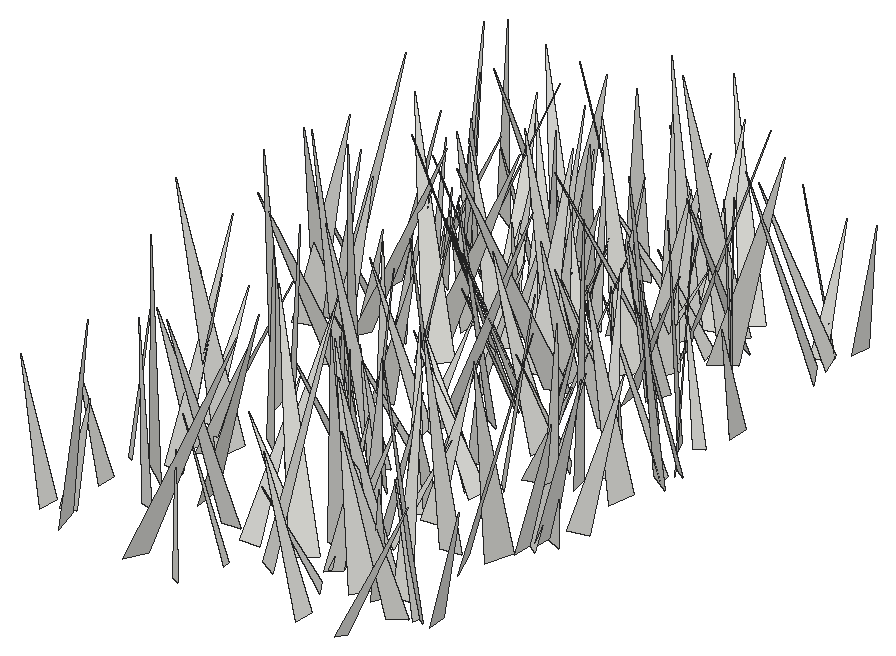
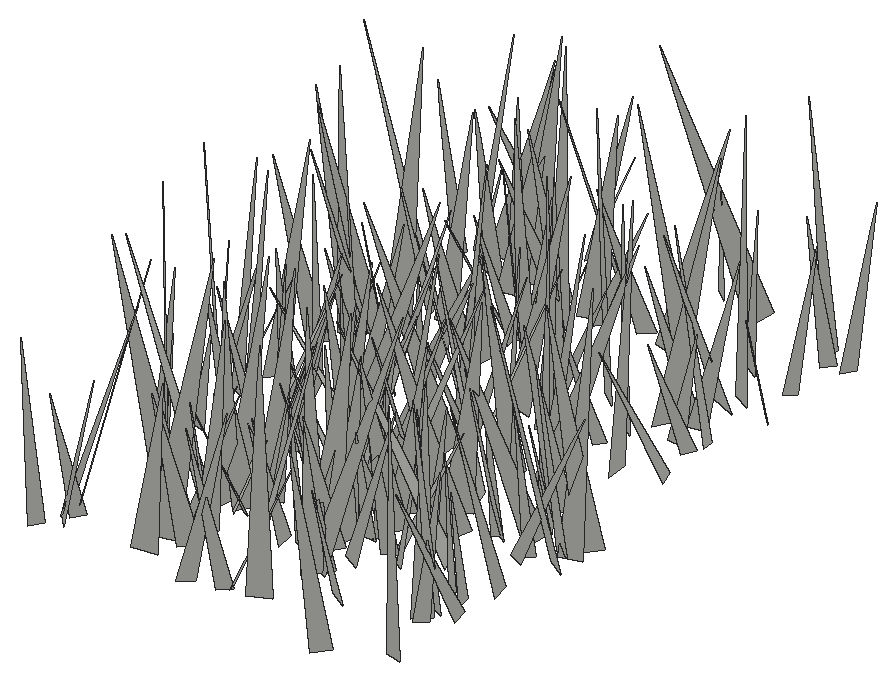
# SketchUp Ruby script. Lengths in inches.
U = 1.inch
M = Sketchup.active_model
def pt(a) = Geom::Point3d.new(a.map { |v| v * U })
def face(e, loops, mat)
  f = e.add_face(loops[0].map { |a| pt(a) })
  loops[1..].each { |l| e.add_face(l.map { |a| pt(a) }).erase! }
  f.material = f.back_material = mat if mat
  f
end
# faces: each face lists its corners as indices into pts; further lists are holes
def faces(e, pts, list, mat = nil) = list.each { |f| face(e, (f[0].is_a?(Array) ? f : [f]).map { |l| l.map { |i| pts[i] } }, mat) }
# xy, xz, yz: faces in a plane at the given z, y or x. An outline is a flat list of corners, or four numbers for a rectangle; further outlines are holes
def ring(l) = l.size == 4 ? [[l[0], l[1]], [l[2], l[1]], [l[2], l[3]], [l[0], l[3]]] : l.each_slice(2).to_a
def flat(e, list, mat, &to3) = list.each { |f| face(e, (f[0].is_a?(Array) ? f : [f]).map { |l| ring(l).map { |u, v| to3.(u, v) } }, mat) }
def xy(e, z, list, mat = nil) = flat(e, list, mat) { |x, y| [x, y, z] }
def xz(e, y, list, mat = nil) = flat(e, list, mat) { |x, z| [x, y, z] }
def yz(e, x, list, mat = nil) = flat(e, list, mat) { |y, z| [x, y, z] }
def lines(e, pts, list) = list.each { |a, b| e.add_line(pt(pts[a]), pt(pts[b])) }
# prism: a flat outline (further loops are holes) pulled along v
def prism(e, loops, v, mat = nil)
  f = face(e, loops, mat); d = Geom::Vector3d.new(v.map { |x| x * U })
  f.pushpull(f.normal.samedirection?(d) ? d.length : -d.length)
end
def box(e, o, s, mat = nil) = prism(e, [[o, [o[0] + s[0], o[1], o[2]], [o[0] + s[0], o[1] + s[1], o[2]], [o[0], o[1] + s[1], o[2]]]], [0, 0, s[2]], mat)
def at(x, y, z, deg = 0) = Geom::Transformation.translation(pt([x, y, z])) * Geom::Transformation.rotation(ORIGIN, Z_AXIS, deg.degrees)
def axes(o, x, y, z) = Geom::Transformation.new([*x, 0, *y, 0, *z, 0, *pt(o).to_a, 1])
def part(name) = M.definitions.add(name)
# library, detail: a bought-in or finely detailed component or shape, given as its bounding box
def library(name, o, s) = part(name).tap { |d| box(d.entities, o, s) }
def detail(e, o, s) = box(e.add_group.entities, o, s)
def put(e, d, t, mat = nil) = e.add_instance(d, t).tap { |i| i.material = mat if mat }
def group(e, t, mat = nil) = e.add_group.tap { |g| g.transformation = t; g.material = mat if mat }.entities
root = M.entities
c1 = part("fur_instance\#9")
p = [[0.8125,0,1.79],[0.67,-0.02,1.48],[0,-0.11,0],[0,0.11,0]]
faces(c1.entities,p,[[0,1,2,3]])
put(root,c1,axes([524.85,163.34,-21.66],[4.20178,-1.75309,2.00996],[-1.5081,-4.65512,-0.90755],[-2.19975,-0.15714,4.46146]))
put(root,c1,axes([525.14,169.86,-21.66],[2.28996,3.33239,0.84649],[3.03653,-2.43723,1.38011],[-1.61271,0.14282,3.80053]))
put(root,c1,axes([523.73,188.04,-21.66],[0.64901,-7.30772,0.94418],[-7.33385,-0.54888,0.79295],[0.71332,1.00569,7.2935]))
put(root,c1,axes([525.92,189.88,-21.66],[-1.33885,-4.31341,0.19295],[-4.24788,1.27969,-0.86785],[-0.77346,0.43835,4.43226]))
put(root,c1,axes([523.4,186.77,-21.66],[4.4224,-5.22883,1.99199],[-5.58659,-4.26873,1.19762],[-0.31423,2.30295,6.7427]))
put(root,c1,axes([525.14,195.22,-21.66],[-3.53887,0.08812,1.47041],[-0.2173,3.75324,-0.74791],[1.45693,0.77383,3.46005]))
put(root,c1,axes([524.35,193.125,-21.66],[5.06172,0.87175,1.3003],[0.68802,-5.19178,0.80241],[-1.40619,0.59773,5.07318]))
put(root,c1,axes([523.75,189.23,-21.66],[-3.45696,-5.56122,4.74392],[-6.59951,4.63089,0.61955],[3.14299,3.60698,6.51874]))
put(root,c1,axes([524.39,187.92,-21.66],[2.41252,4.65389,1.89869],[5.02303,-2.30836,-0.72433],[-0.1815,-2.02404,5.19175]))
put(root,c1,axes([524.4,202.02,-21.66],[-2.31612,-6.1908,2.36322],[-6.27799,2.85121,1.3163],[2.12077,1.67923,6.47748]))
put(root,c1,axes([524.36,196.52,-21.66],[4.0884,0.15219,0.34801],[0.0557,-3.96154,1.07814],[-0.37573,1.0688,3.94662]))
put(root,c1,axes([525.62,198.18,-21.66],[3.23004,-2.47849,1.2151],[-2.38486,-3.44753,-0.69249],[-1.3899,0.15559,4.01205]))
put(root,c1,axes([527.1,174.92,-21.66],[-1.4583,4.1794,0.64732],[4.14586,1.27741,1.09233],[-0.83566,-0.95598,4.28962]))
put(root,c1,axes([526.01,196.63,-21.66],[2.58836,6.22661,1.98748],[6.38761,-2.86286,0.6503],[-1.38536,-1.56644,6.71174]))
put(root,c1,axes([525.71,167.12,-21.66],[-3.46561,0.71078,2.1355],[1.4755,3.67824,1.17025],[1.69955,-1.74395,3.33859]))
put(root,c1,axes([526.01,175.26,-21.66],[-2.24412,3.20659,0.81725],[3.00578,2.38826,-1.11699],[1.38398,0.01256,3.75108]))
put(root,c1,axes([526.45,186.17,-21.66],[2.93854,2.24557,1.05284],[2.03507,-3.11619,0.96641],[-1.41759,0.18132,3.56983]))
put(root,c1,axes([525.23,178.12,-21.66],[4.11341,0.99659,0.14821],[0.94897,-4.04143,0.83763],[-0.33855,0.78037,4.1487]))
put(root,c1,axes([527.24,173.08,-21.66],[2.70621,-3.86796,1.26709],[-3.69816,-2.97221,-1.17466],[-1.70008,0.30833,4.57219]))
put(root,c1,axes([525.55,189.17,-21.66],[0.50493,-3.90237,0.56248],[-3.75126,-0.30094,1.27958],[1.21364,0.69337,3.72104]))
put(root,c1,axes([527.2,195.37,-21.66],[3.68214,4.39884,2.0354],[4.4735,-4.06815,0.69917],[-1.86561,-1.07294,5.69378]))
put(root,c1,axes([526.01,163.5625,-21.66],[2.52401,-3.24586,0.70539],[-3.32076,-2.44552,0.62916],[0.07602,0.94215,4.0633]))
put(root,c1,axes([526.38,194.6,-21.66],[-1.07299,-3.39329,1.1863],[-3.30809,1.41653,1.05972],[1.4065,0.74301,3.39746]))
put(root,c1,axes([525.87,197.8125,-21.66],[5.72206,-2.67718,0.30846],[-2.55509,-5.6197,-1.37653],[-0.85672,-1.12072,6.16558]))
put(root,c1,axes([525.7,174.0625,-21.66],[5.69454,1.71793,1.14191],[1.95584,-5.5622,-1.38552],[-0.6557,-1.67144,5.78441]))
put(root,c1,axes([527.66,170.34,-21.66],[1.84381,6.83005,0.32521],[6.75707,-1.87158,0.99709],[-1.04756,-0.05069,7.00393]))
put(root,c1,axes([528.85,173.62,-21.66],[-7.80525,1.8691,2.4402],[2.24771,8.01322,1.05174],[2.09664,-1.63243,7.95672]))
put(root,c1,axes([527.66,179.24,-21.66],[-7.27615,-1.41209,3.18772],[-1.2687,7.94356,0.62294],[3.24745,-0.06052,7.38568]))
put(root,c1,axes([527.25,169.3,-21.66],[-3.84702,-6.56229,2.86732],[-6.71624,4.43571,1.14075],[2.48541,1.82909,7.52076]))
put(root,c1,axes([527.22,184.41,-21.66],[4.47757,-3.00826,2.16701],[-3.51648,-4.52249,0.98776],[-1.1747,2.07164,5.30307]))
put(root,c1,axes([526.73,162.48,-21.66],[6.91292,1.02767,1.79019],[1.3308,-7.00178,-1.11957],[-1.57792,-1.40299,6.89863]))
put(root,c1,axes([529.01,166.37,-21.66],[1.89742,4.59885,2.05217],[4.78177,-2.33318,0.8074],[-1.57969,-1.53878,4.90894]))
put(root,c1,axes([529.65,182.67,-21.66],[0.11863,-7.1905,0.64579],[-7.08435,-0.24031,-1.37429],[-1.39009,0.61104,7.05894]))
put(root,c1,axes([526.29,187.75,-21.66],[6.61677,-1.08212,0.53072],[-1.15649,-6.53431,1.0953],[-0.3394,1.16883,6.6146]))
put(root,c1,axes([531.11,193.3,-21.66],[-3.78552,-3.06993,0.30173],[-3.01727,3.58565,-1.37288],[-0.64154,1.25071,4.67652]))
put(root,c1,axes([528.02,188.53,-21.66],[2.95558,3.83246,1.3061],[4.0436,-2.87668,-0.7093],[-0.20723,-1.47175,4.78749]))
put(root,c1,axes([528.28,188.51,-21.66],[0.50859,-3.54434,0.97529],[-3.61365,-0.30136,0.78924],[0.67458,1.05784,3.49258]))
put(root,c1,axes([528.72,184.1,-21.66],[6.72646,1.81373,2.96578],[2.30607,-7.16166,-0.85049],[-2.60144,-1.65881,6.91459]))
put(root,c1,axes([527.8,203.87,-21.66],[3.51302,-4.23345,1.0034],[-4.35037,-3.40123,0.88101],[0.05668,1.33409,5.43021]))
put(root,c1,axes([527.8,172.63,-21.66],[3.87779,-2.1954,0.31482],[-2.2129,-3.78759,0.8446],[0.14815,0.88911,4.37535]))
put(root,c1,axes([531.5,180.16,-21.66],[-7.85501,-1.13743,1.66782],[-1.3997,7.89692,-1.20666],[1.45472,1.45652,7.84468]))
put(root,c1,axes([531.43,187.85,-21.66],[-4.74257,5.72398,1.5327],[5.90767,4.72004,0.65254],[0.46105,-1.60076,7.40474]))
put(root,c1,axes([530.96,183.72,-21.66],[-3.9297,0.38452,0.60241],[0.18265,3.7953,-1.23109],[0.69093,1.18368,3.75164]))
put(root,c1,axes([530.55,198.99,-21.66],[1.48106,4.37962,0.44895],[4.22706,-1.54701,1.14671],[-1.23071,-0.04293,4.4788]))
put(root,c1,axes([530.28,191.71,-21.66],[3.55115,-1.15094,1.45453],[-0.93925,-3.82501,-0.73353],[-1.59941,-0.30919,3.66022]))
put(root,c1,axes([530.29,194.23,-21.66],[-2.2334,-3.12116,0.78897],[-3.02774,2.36275,0.77617],[1.09405,0.16724,3.75863]))
put(root,c1,axes([530.01,175.49,-21.66],[-3.26006,-5.04679,2.60885],[-5.29814,3.78652,0.70434],[2.05082,1.75965,5.96674]))
put(root,c1,axes([530.68,187.12,-21.66],[1.32341,3.79294,0.4756],[3.74321,-1.38791,0.65276],[-0.77522,-0.22654,3.9638]))
put(root,c1,axes([530.23,177.4375,-21.66],[-1.29453,3.3269,0.92168],[3.25121,1.50588,-0.8692],[1.16077,-0.50757,3.46245]))
put(root,c1,axes([528.58,192.16,-21.66],[7.17048,3.0592,0.30714],[3.02615,-7.16002,0.66735],[-0.54355,0.49421,7.76718]))
put(root,c1,axes([532.53,195.46,-21.66],[-2.18314,-4.32344,1.23175],[-4.48368,1.99494,-0.94459],[-0.32548,1.51774,4.75036]))
put(root,c1,axes([533.52,197.1,-21.66],[-2.92587,-7.18113,1.16279],[-7.26033,2.80394,-0.95233],[-0.45638,1.43204,7.69561]))
put(root,c1,axes([533.04,191.04,-21.66],[-4.86777,3.35697,1.6535],[3.6105,4.92638,0.62739],[0.98366,-1.46972,5.8797]))
put(root,c1,axes([532.75,191.42,-21.66],[-3.90742,5.66938,0.63215],[5.60395,3.95813,-0.85923],[1.06639,-0.02677,6.83166]))
put(root,c1,axes([531.41,193.58,-21.66],[-0.36242,4.3186,2.109],[4.6668,0.82166,-0.88056],[1.14855,-1.97588,4.24338]))
put(root,c1,axes([534.96,188.96,-21.66],[-5.01465,-5.39389,0.78065],[-5.43536,4.87162,-1.25473],[-0.40033,1.42249,7.25716]))
put(root,c1,axes([529.86,189.77,-21.66],[6.60673,-3.01857,0.44503],[-3.04917,-6.49303,1.22551],[0.11127,1.29906,7.15953]))
put(root,c1,axes([533.4,192.93,-21.66],[-0.37252,4.33667,0.3989],[4.3129,0.31185,0.63743],[-0.60398,-0.44793,4.30572]))
put(root,c1,axes([533.8,167.49,-21.66],[-0.89834,-6.55906,1.37521],[-6.65422,0.70817,-0.96916],[-0.7961,1.48213,6.54897]))
put(root,c1,axes([531.47,185.8,-21.66],[5.91305,2.63208,1.30513],[2.84881,-5.85376,-1.10147],[-0.71801,-1.54954,6.37799]))
put(root,c1,axes([534.12,176.74,-21.66],[-0.56318,-3.80765,0.20803],[-3.75255,0.51599,-0.71463],[-0.67806,0.30692,3.78215]))
put(root,c1,axes([533.07,192.55,-21.66],[3.93197,-0.07434,1.3447],[0.21137,-4.06439,-0.84276],[-1.33006,-0.86567,3.84131]))
put(root,c1,axes([530.95,169.11,-21.66],[7.51831,-0.309,0.51299],[-0.23256,-7.46002,-1.08516],[-0.55186,-1.06592,7.446]))
put(root,c1,axes([533.35,189.47,-21.66],[-1.89071,3.52857,0.74513],[3.44423,2.01617,-0.80816],[1.06925,-0.25501,3.92077]))
put(root,c1,axes([532.84,173.45,-21.66],[-4.52397,-6.09316,3.51067],[-6.34353,5.33763,1.08955],[3.03497,2.07386,7.51038]))
put(root,c1,axes([533.15,191.66,-21.66],[3.71678,-0.58843,1.31141],[-0.99782,-3.67326,1.17982],[-1.0346,1.42876,3.57333]))
put(root,c1,axes([535.73,193.66,-21.66],[-3.99948,7.12267,1.32626],[7.23474,3.8453,1.16596],[-0.38726,-1.72292,8.0851]))
put(root,c1,axes([531.8,182.66,-21.66],[3.60736,-4.41491,0.21347],[-4.38405,-3.53869,0.89879],[0.56311,0.73233,5.62998]))
put(root,c1,axes([535.46,192.37,-21.66],[-3.34888,5.66427,0.75226],[5.70524,3.26636,0.80369],[-0.31635,-1.05439,6.53093]))
put(root,c1,axes([533.98,194.94,-21.66],[-3.10832,3.75001,0.92239],[3.63037,3.24121,-0.94342],[1.31674,-0.08395,4.77852]))
put(root,c1,axes([535.49,181.71,-21.66],[-5.30182,-0.75056,0.88287],[-0.65483,5.35184,0.61739],[0.95603,-0.49663,5.31898]))
put(root,c1,axes([536.19,164.09,-21.66],[-3.92472,-1.58946,0.29836],[-1.61245,3.78584,-1.04222],[-0.12416,1.07696,4.10409]))
put(root,c1,axes([532.82,197.1,-21.66],[2.13927,-3.81253,0.27989],[-3.71667,-1.99926,1.17453],[0.89447,0.81104,4.21098]))
put(root,c1,axes([533.46,178.13,-21.66],[0.2783,-5.0487,0.14304],[-4.93686,-0.24166,1.07529],[1.0664,0.19877,4.94071]))
put(root,c1,axes([535.49,194.62,-21.66],[-2.59622,-3.87524,1.56211],[-4.17566,2.47102,-0.8099],[0.14666,1.75346,4.59368]))
put(root,c1,axes([535.91,177.25,-21.66],[-0.62718,-6.98929,2.39617],[-7.29856,0.2117,-1.29283],[-1.15016,2.46782,6.89725]))
put(root,c1,axes([535.15,161.12,-21.66],[1.49909,3.09185,1.25062],[3.12666,-1.78006,0.6529],[-1.16087,-0.8017,3.3735]))
put(root,c1,axes([536.6875,198.15,-21.66],[-5.72763,-4.55632,1.57593],[-4.80185,5.61014,-1.23206],[0.43111,1.95337,7.21442]))
put(root,c1,axes([535.74,180.05,-21.66],[-3.80651,-3.12707,0.03174],[-3.06593,3.74155,0.93273],[0.61617,-0.70095,4.83716]))
put(root,c1,axes([535.66,201.57,-21.66],[-3.34335,-1.51871,0.13226],[-1.40215,3.18862,1.16988],[0.59829,-1.01398,3.48078]))
put(root,c1,axes([531.91,161.85,-21.66],[7.97011,-1.5942,0.50435],[-1.65185,-7.88792,1.1707],[-0.25934,1.24806,8.04323]))
put(root,c1,axes([533.93,201.4,-21.66],[1.85268,-6.56464,1.39244],[-6.70428,-1.74747,0.68181],[0.2934,1.52239,6.78691]))
put(root,c1,axes([534.05,193.71,-21.66],[6.7511,0.38921,2.10678],[0.68602,-6.99103,-0.90679],[-2.02963,-1.06837,6.70124]))
put(root,c1,axes([536.55,187.47,-21.66],[-2.94659,-4.28728,0.79485],[-4.35538,2.84813,-0.78348],[-0.2081,1.09651,5.14289]))
put(root,c1,axes([533.1875,197.65,-21.66],[6.03142,-3.81553,0.06105],[-3.78285,-5.99326,-0.84318],[-0.50203,-0.68018,7.08699]))
put(root,c1,axes([535.51,195.89,-21.66],[1.56469,4.5597,1.40699],[4.65343,-1.78584,0.61247],[-1.05645,-1.11294,4.78163]))
put(root,c1,axes([536.89,175.51,-21.66],[0.66208,3.60921,1.19442],[3.54519,-1.02396,1.12897],[-1.37285,-0.90361,3.49144]))
put(root,c1,axes([534.85,186.93,-21.66],[2.48119,3.58815,0.88423],[3.68479,-2.32113,-0.92071],[0.2811,-1.24521,4.2642]))
put(root,c1,axes([536.8,191.47,-21.66],[-6.28621,2.90163,2.83322],[3.4688,6.55463,0.9835],[2.10096,-2.14018,6.85337]))
put(root,c1,axes([535.33,181.89,-21.66],[0.85166,3.52496,0.51911],[3.494,-0.72175,-0.83136],[0.69768,-0.68839,3.5298]))
put(root,c1,axes([535.7,166.67,-21.66],[-1.59343,4.55905,1.08338],[4.45907,1.82697,-1.12985],[1.44061,-0.61229,4.69546]))
put(root,c1,axes([535.42,174.43,-21.66],[5.69502,0.05498,1.49404],[0.36012,-5.7612,-1.16071],[-1.45103,-1.21405,5.57575]))
put(root,c1,axes([537.71,186.48,-21.66],[-2.11494,-3.26023,0.3236],[-3.25153,2.04149,-0.68318],[-0.40176,0.64034,3.82562]))
put(root,c1,axes([534.41,194.85,-21.66],[4.26627,1.55205,0.05399],[1.49304,-4.05567,-1.39111],[0.42732,-1.32496,4.32143]))
put(root,c1,axes([537.6875,184.46,-21.66],[-3.61019,-4.99925,2.09321],[-5.40705,3.49453,-0.97958],[0.37125,2.28107,6.08822]))
put(root,c1,axes([537.33,171.78,-21.66],[-3.18847,2.06393,0.29466],[1.98964,3.17316,-0.69666],[0.62286,0.42918,3.73374]))
put(root,c1,axes([535.83,192.47,-21.66],[0.28341,4.29415,2.46111],[4.89058,0.13603,-0.80051],[0.76092,-2.47364,4.22839]))
put(root,c1,axes([536.58,195.93,-21.66],[-4.01234,0.85775,1.7856],[0.34464,4.27421,-1.27879],[1.95072,1.00913,3.89863]))
put(root,c1,axes([536.22,190.13,-21.66],[-1.99924,6.11191,2.2816],[6.3463,2.375,-0.80119],[1.51181,-1.88733,6.38047]))
put(root,c1,axes([538.34,167.74,-21.66],[-3.99734,1.08155,0.32432],[1.12476,3.91891,0.79421],[0.09918,-0.85212,4.0642]))
put(root,c1,axes([536.63,188.74,-21.66],[3.04717,-2.22298,0.43436],[-2.028,-3.00193,-1.13631],[-1.00873,-0.67996,3.59662]))
put(root,c1,axes([536.15,176.23,-21.66],[-4.08433,-4.26667,3.28401],[-4.58243,4.91876,0.69141],[2.82675,1.80893,5.86585]))
put(root,c1,axes([538.15,189.41,-21.66],[0.33917,-8.30019,0.61155],[-8.21231,-0.43312,-1.32383],[-1.35096,0.54903,8.20095]))
put(root,c1,axes([535.84,201.86,-21.66],[1.71183,-4.04593,1.56999],[-4.29437,-1.33542,1.2409],[0.62675,1.9005,4.21427]))
put(root,c1,axes([538,202.4375,-21.66],[-4.52682,2.09063,1.69581],[2.46981,4.54531,0.98938],[1.07078,-1.64562,4.88712]))
put(root,c1,axes([538.89,167.25,-21.66],[2.27452,-5.56414,4.58515],[-6.58849,-3.55674,-1.04785],[-2.92831,3.68058,5.91904]))
put(root,c1,axes([537.34,180.47,-21.66],[-4.05006,-5.82532,2.03849],[-5.82326,4.4146,1.04584],[2.04438,1.03428,7.01738]))
put(root,c1,axes([538.63,186.6875,-21.66],[-4.50054,-5.78959,0.45114],[-5.68851,4.51005,1.13049],[1.1678,-0.3432,7.24542]))
put(root,c1,axes([537.59,175.63,-21.66],[-1.86728,-3.21645,1.13397],[-3.16749,2.11482,0.78275],[1.26429,0.54787,3.63587]))
put(root,c1,axes([539.47,185.64,-21.66],[-1.836,-5.36618,0.72675],[-5.38286,1.72484,-0.86298],[-0.59066,0.96126,5.60554]))
put(root,c1,axes([535.95,182.86,-21.66],[7.40622,-0.19557,0.80001],[-0.28757,-7.3972,0.85392],[-0.77173,0.87956,7.35943]))
put(root,c1,axes([538.14,190.54,-21.66],[-4.48343,0.78051,2.64752],[1.64873,4.80743,1.37477],[2.21365,-1.99978,4.33824]))
put(root,c1,axes([539.57,193.85,-21.66],[1.87721,3.55983,2.07479],[3.45548,-2.60202,1.33802],[-2.2443,-1.02868,3.79553]))
put(root,c1,axes([538.09,165.1875,-21.66],[3.95249,6.61953,0.92655],[6.54498,-4.05132,1.02412],[-1.35642,-0.25967,7.64143]))
put(root,c1,axes([540.08,198.125,-21.66],[-7.50799,1.69583,1.59774],[1.55933,7.66276,-0.80567],[1.73121,0.45255,7.65484]))
put(root,c1,axes([539.26,170.23,-21.66],[-4.67336,-1.61213,2.14084],[-2.03116,4.93814,-0.71533],[1.7483,1.42769,4.89159]))
put(root,c1,axes([538.5,188.84,-21.66],[3.62249,2.81644,0.55831],[2.6251,-3.61284,1.19278],[-1.16313,0.61769,4.43081]))
put(root,c1,axes([539.93,193.14,-21.66],[-5.03128,5.10175,2.45438],[5.52933,5.13327,0.66454],[1.21582,-2.23324,7.13442]))
put(root,c1,axes([541.29,178.43,-21.66],[-3.62089,2.64212,0.01483],[2.58278,3.53416,0.96476],[-0.55698,-0.78788,4.37731]))
put(root,c1,axes([540.94,194.83,-21.66],[-5.31992,-4.92486,0.01845],[-4.88394,5.27914,0.91325],[0.63384,-0.65774,7.19179]))
put(root,c1,axes([538.33,199.66,-21.66],[3.90059,1.73334,0.99556],[1.91928,-3.85762,-0.80331],[-0.55855,-1.15086,4.19211]))
put(root,c1,axes([540.46,174.45,-21.66],[-4.55116,2.07867,0.64916],[1.93391,4.54938,-1.00919],[1.00113,0.66152,4.90056]))
put(root,c1,axes([541.84,178.11,-21.66],[-4.37284,2.10544,0.41102],[2.13916,4.20984,1.19366],[-0.16073,-1.25217,4.70423]))
put(root,c1,axes([541.74,201.27,-21.66],[-2.77056,6.19265,0.76015],[6.19361,2.62958,1.15202],[-0.75223,-1.15721,6.68563]))
put(root,c1,axes([540.23,199.38,-21.66],[-3.17134,4.85922,0.78552],[4.77597,3.26378,-0.90795],[1.19131,-0.14895,5.73106]))
put(root,c1,axes([541.85,168.15,-21.66],[-4.80614,1.67739,0.07303],[1.63862,4.73444,-0.90443],[0.36591,0.83033,5.00945]))
put(root,c1,axes([538.64,178.56,-21.66],[3.81482,2.67004,0.71919],[2.75746,-3.58156,-1.32965],[0.20681,-1.49748,4.4625]))
put(root,c1,axes([539.56,180.73,-21.66],[0.99148,-3.49866,0.36174],[-3.47594,-0.91715,0.65665],[0.53788,0.52224,3.57665]))
put(root,c1,axes([541.49,183.98,-21.66],[-5.54142,2.04017,2.02802],[2.50487,5.58649,1.22443],[1.41448,-1.90035,5.77671]))
put(root,c1,axes([539.79,169.07,-21.66],[-0.40221,-7.56998,1.93164],[-7.73436,0.65878,0.97125],[1.10251,1.85984,7.51818]))
put(root,c1,axes([541.58,165.3,-21.66],[-3.32799,-2.15223,0.18164],[-2.02775,3.22824,1.09879],[0.74386,-0.82886,3.80792]))
put(root,c1,axes([541.56,194.41,-21.66],[-6.82221,1.72842,2.33339],[1.55801,7.20655,-0.7829],[2.45045,0.23004,6.99407]))
put(root,c1,axes([541.84,199.6,-21.66],[2.92408,-7.38877,2.72238],[-7.56214,-3.44459,-1.22649],[-2.19528,2.02396,7.85111]))
put(root,c1,axes([540.09,171.35,-21.66],[0.10364,-5.95888,1.80759],[-6.13378,0.21397,1.05707],[1.07352,1.79787,5.86529]))
put(root,c1,axes([540.71,171.65,-21.66],[4.041,0.55824,1.1889],[0.26805,-4.11576,1.02147],[-1.28579,0.89645,3.94942]))
put(root,c1,axes([541.94,197.39,-21.66],[-3.71284,-0.24914,0.82183],[0.046,3.58403,1.29433],[0.85753,-1.27095,3.48884]))
put(root,c1,axes([540.91,175.34,-21.66],[3.64038,-1.44849,0.64201],[-1.22649,-3.59476,-1.15586],[-1.003,-0.8615,3.74359]))
put(root,c1,axes([539.97,194.91,-21.66],[2.36408,2.77163,0.06713],[2.67068,-2.25294,-1.03299],[0.74428,-0.71945,3.49339]))
put(root,c1,axes([542.6,188.58,-21.66],[-4.67386,-0.0885,1.27111],[0.2568,4.66814,1.26925],[1.24804,-1.29194,4.49909]))
put(root,c1,axes([540.37,194.45,-21.66],[-2.5167,4.57974,3.46384],[4.9953,3.61127,-1.14527],[2.83182,-2.30014,5.09864]))
put(root,c1,axes([542.87,162.23,-21.66],[-4.85785,0.78834,1.37895],[1.02249,4.94749,0.77364],[1.21552,-1.0112,4.86021]))
put(root,c1,axes([541.01,167.04,-21.66],[4.40781,-2.35415,1.32075],[-2.57038,-4.43283,0.67704],[-0.82436,1.23418,4.95101]))
put(root,c1,axes([542.6875,188.03,-21.66],[1.51534,-5.37644,0.92666],[-5.31705,-1.67082,-0.99923],[-1.22223,0.60275,5.49581]))
put(root,c1,axes([543.7,187.68,-21.66],[-3.57996,-1.2077,0.30439],[-1.24532,3.48547,-0.8173],[0.0195,0.87192,3.68872]))
put(root,c1,axes([541.07,167.27,-21.66],[4.54007,-1.04122,1.07478],[-1.33062,-4.37982,1.37772],[-0.68465,1.60765,4.44952]))
put(root,c1,axes([541.59,184.15,-21.66],[4.07971,3.91858,0.07723],[3.79656,-3.97882,1.32677],[-0.97331,0.90496,5.499]))
put(root,c1,axes([542.36,179.5625,-21.66],[3.86177,3.77021,1.4507],[3.73701,-4.09632,0.69796],[-1.5342,-0.48777,5.35169]))
put(root,c1,axes([541.75,174.29,-21.66],[-1.54169,4.36128,2.00643],[4.43238,2.10262,-1.16464],[1.84406,-1.40768,4.47674]))
put(root,c1,axes([541.65,171.11,-21.66],[1.90499,3.12749,0.05078],[3.06447,-1.8542,-0.76405],[0.62675,-0.43991,3.5814]))
put(root,c1,axes([543.7,166.33,-21.66],[-5.4764,4.5647,2.90915],[5.14181,5.68019,0.76664],[1.69155,-2.48788,7.08799]))
put(root,c1,axes([542.74,192.14,-21.66],[4.44508,-4.04211,0.97735],[-3.87336,-4.54492,-1.18043],[-1.51359,-0.24009,5.89101]))
put(root,c1,axes([542.73,199.13,-21.66],[-1.67702,-6.45132,0.05531],[-6.32349,1.655,1.30744],[1.27907,-0.27646,6.53625]))
put(root,c1,axes([543.75,183.47,-21.66],[-3.41692,-2.65793,0.41527],[-2.50813,3.39027,1.06197],[0.9728,-0.5949,4.19669]))
put(root,c1,axes([543.88,167.88,-21.66],[2.81422,-5.9892,1.8303],[-5.99838,-3.15452,-1.09945],[-1.79999,1.14839,6.52546]))
put(root,c1,axes([540.91,196.57,-21.66],[7.89024,2.57718,0.73013],[2.64489,-7.85516,-0.85554],[-0.42369,-1.04189,8.25626]))
put(root,c1,axes([541.65,191.01,-21.66],[5.27208,0.02621,0.0042],[0.02652,-5.23568,-0.61848],[-0.0011,-0.61849,5.23574]))
put(root,c1,axes([544.51,172.5,-21.66],[-0.07394,-6.12578,2.47714],[-6.56947,-0.19789,-0.68546],[-0.70961,2.47033,6.08776]))
put(root,c1,axes([543.55,190.71,-21.66],[-3.953,-6.85404,2.35159],[-6.87911,4.39144,1.23577],[2.27722,1.36799,7.81517]))
put(root,c1,axes([544.67,195.87,-21.66],[-3.59286,-3.26733,2.03566],[-3.70516,3.69058,-0.61592],[1.04455,1.85261,4.81713]))
put(root,c1,axes([545.33,182.19,-21.66],[-6.71268,-1.89599,2.76742],[-2.51748,6.93875,-1.3526],[2.21714,2.13833,6.8429]))
put(root,c1,axes([543.06,181.01,-21.66],[3.00481,-2.76961,0.12717],[-2.71494,-2.90128,0.96303],[0.56213,0.79222,3.97142]))
put(root,c1,axes([545.77,185.09,-21.66],[-4.75488,-0.89522,1.48594],[-1.16705,4.85843,-0.80746],[1.28353,1.10117,4.77057]))
put(root,c1,axes([545.71,166.97,-21.66],[0.35449,6.1752,1.09899],[6.2119,-0.49795,0.79425],[-0.86782,-1.04187,6.13416]))
put(root,c1,axes([546.05,183.73,-21.66],[-0.40963,5.6712,0.85204],[5.69515,0.30195,0.72827],[-0.67361,-0.89587,5.63914]))
put(root,c1,axes([543.1875,196.99,-21.66],[6.11915,-4.70581,1.11272],[-4.83462,-5.98952,1.25659],[-0.09634,1.67568,7.61641]))
put(root,c1,axes([546.8,165.16,-21.66],[0.96308,-5.75121,1.64983],[-5.7805,-1.32563,-1.24675],[-1.54408,1.37555,5.69645]))
put(root,c1,axes([544.76,166.27,-21.66],[3.91329,-2.80057,0.16354],[-2.76188,-3.89534,-0.61821],[-0.49189,-0.40864,4.7723]))
put(root,c1,axes([547.09,201.38,-21.66],[2.56501,3.25674,2.5986],[3.3721,-3.41499,0.95138],[-2.44704,-1.29222,4.03491]))
put(root,c1,axes([546.9,188.73,-21.66],[-5.34444,-2.84039,2.21318],[-3.30562,5.4408,-0.99979],[1.42788,1.96442,5.96919]))
put(root,c1,axes([548.45,185.5,-21.66],[-4.94313,-1.68267,0.02369],[-1.64372,4.81198,-1.18726],[-0.36076,1.13137,5.08492]))
put(root,c1,axes([547.63,165.95,-21.66],[-4.59653,-5.39297,2.39685],[-5.86856,4.49796,-1.13384],[0.62378,2.57709,6.99476]))
put(root,c1,axes([547.69,165.67,-21.66],[-3.7674,-0.4134,0.34529],[-0.49063,3.64055,-0.99453],[0.22227,1.02903,3.6572]))
put(root,c1,axes([547.5,200.63,-21.66],[-5.8236,-1.97497,1.08531],[-1.72724,5.8434,1.36532],[1.44743,-0.9731,5.99589]))
put(root,c1,axes([547.8,189.21,-21.66],[-0.43735,3.78387,0.74816],[3.7266,0.2203,1.06426],[-0.99494,-0.83814,3.65736]))
put(root,c1,axes([547.68,199.11,-21.66],[-5.81163,-3.8947,1.27527],[-3.71182,5.94036,1.22659],[1.73708,-0.33677,6.88761]))
put(root,c1,axes([546.72,200.59,-21.66],[-2.21972,3.26489,1.22418],[3.2229,2.47495,-0.75684],[1.3308,-0.54808,3.87477]))
put(root,c1,axes([545.625,161.92,-21.66],[4.34496,-0.35551,0.43941],[-0.4633,-4.19131,1.19014],[-0.32376,1.22666,4.19388]))
put(root,c1,axes([548.75,186.47,-21.66],[-3.27995,-3.84872,1.10692],[-4.00472,3.15616,-0.89264],[0.01123,1.42196,4.97734]))
put(root,c1,axes([546.94,173.52,-21.66],[6.05759,-4.04132,1.47541],[-3.82561,-6.22554,-1.34569],[-1.96821,-0.33746,7.15653]))
put(root,c1,axes([548.03,182.43,-21.66],[-6.01027,1.97565,2.91231],[2.62602,6.35479,1.10849],[2.3428,-2.05464,6.22879]))
put(root,c1,axes([547.34,192.36,-21.66],[6.08028,3.66314,2.96745],[4.34842,-6.22849,-1.22118],[-1.82087,-2.64225,6.99265]))
put(root,c1,axes([545.92,171.76,-21.66],[7.78659,2.72532,1.24866],[2.87625,-7.77148,-0.97412],[-0.84485,-1.33952,8.19204]))
put(root,c1,axes([547.33,174.98,-21.66],[6.67173,1.075,1.66778],[0.88806,-6.84957,0.86244],[-1.77439,0.61387,6.70252]))
put(root,c1,axes([548.48,185.03,-21.66],[-3.10043,-5.65859,2.0595],[-5.81568,3.41455,0.62657],[1.56175,1.48157,6.42182]))
put(root,c1,axes([547.35,175.63,-21.66],[2.91311,4.64162,1.0633],[4.76072,-2.81168,-0.76908],[0.10392,-1.30816,5.4258]))
put(root,c1,axes([547.78,176.6875,-21.66],[-1.4348,-7.0433,2.45033],[-7.23254,1.92235,1.29061],[1.81726,2.08982,7.07114]))
put(root,c1,axes([548.05,186.97,-21.66],[-5.21121,-4.35385,3.58957],[-4.50193,6.15376,0.92827],[3.40202,1.4741,6.72689]))
put(root,c1,axes([547.91,202.6,-21.66],[4.83385,-1.43847,0.54232],[-1.36908,-4.84202,-0.64023],[-0.69925,-0.46374,5.00254]))
put(root,c1,axes([548.45,191.67,-21.66],[4.29129,-1.7599,0.57931],[-1.53313,-4.1935,-1.38278],[-1.04037,-1.07949,4.42723]))
put(root,c1,axes([547.6875,176.39,-21.66],[6.64533,-1.36705,0.39109],[-1.31179,-6.61549,-0.83466],[-0.54862,-0.74069,6.73295]))
put(root,c1,axes([548.49,178.23,-21.66],[3.34726,-4.07819,1.53745],[-4.35777,-3.09938,1.26621],[0.07255,1.99042,5.12177]))
put(root,c1,axes([548.64,166.15,-21.66],[4.67229,-0.63233,0.28263],[-0.57173,-4.60903,-0.86025],[-0.39095,-0.81674,4.63574]))
